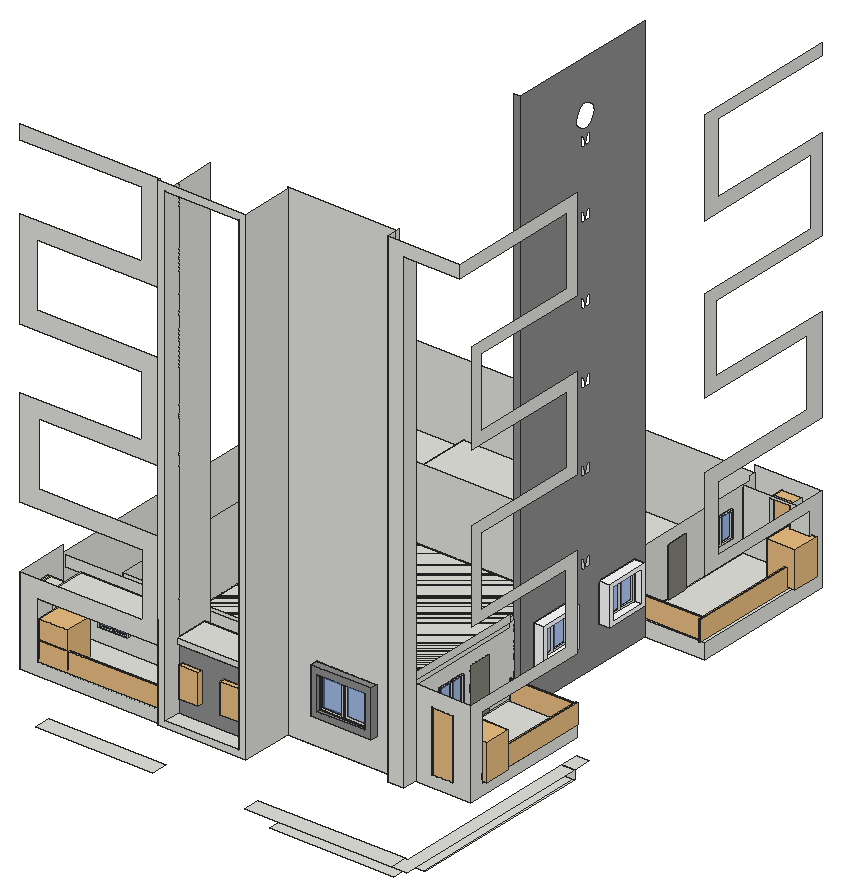
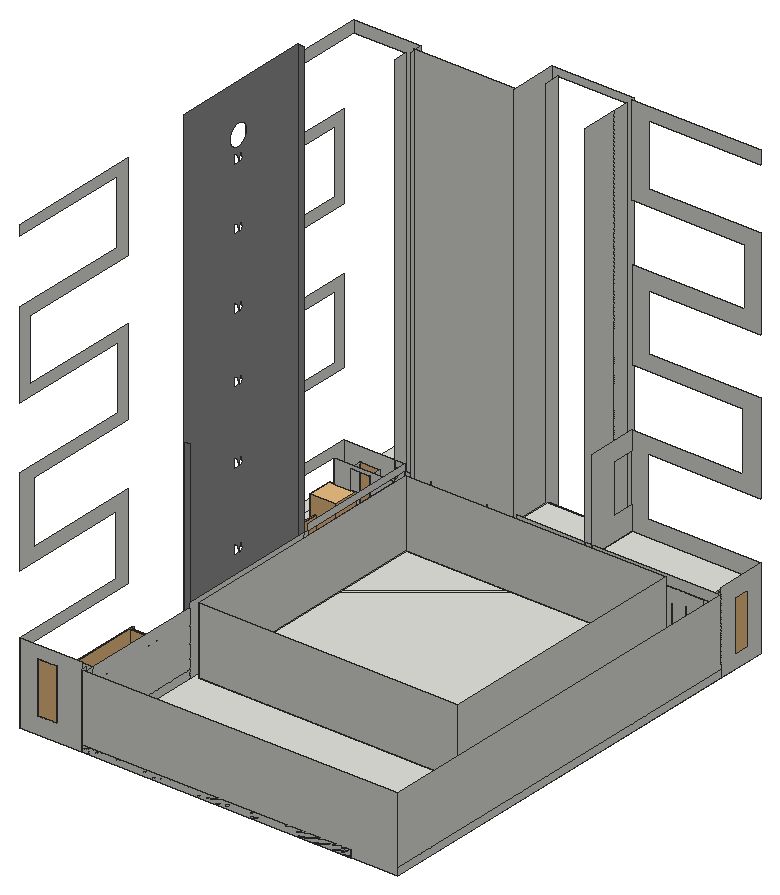
# SketchUp Ruby script. Lengths in inches.
U = 1.inch
M = Sketchup.active_model
def pt(a) = Geom::Point3d.new(a.map { |v| v * U })
def face(e, loops, mat)
  f = e.add_face(loops[0].map { |a| pt(a) })
  loops[1..].each { |l| e.add_face(l.map { |a| pt(a) }).erase! }
  f.material = f.back_material = mat if mat
  f
end
# faces: each face lists its corners as indices into pts; further lists are holes
def faces(e, pts, list, mat = nil) = list.each { |f| face(e, (f[0].is_a?(Array) ? f : [f]).map { |l| l.map { |i| pts[i] } }, mat) }
# xy, xz, yz: faces in a plane at the given z, y or x. An outline is a flat list of corners, or four numbers for a rectangle; further outlines are holes
def ring(l) = l.size == 4 ? [[l[0], l[1]], [l[2], l[1]], [l[2], l[3]], [l[0], l[3]]] : l.each_slice(2).to_a
def flat(e, list, mat, &to3) = list.each { |f| face(e, (f[0].is_a?(Array) ? f : [f]).map { |l| ring(l).map { |u, v| to3.(u, v) } }, mat) }
def xy(e, z, list, mat = nil) = flat(e, list, mat) { |x, y| [x, y, z] }
def xz(e, y, list, mat = nil) = flat(e, list, mat) { |x, z| [x, y, z] }
def yz(e, x, list, mat = nil) = flat(e, list, mat) { |y, z| [x, y, z] }
def lines(e, pts, list) = list.each { |a, b| e.add_line(pt(pts[a]), pt(pts[b])) }
# prism: a flat outline (further loops are holes) pulled along v
def prism(e, loops, v, mat = nil)
  f = face(e, loops, mat); d = Geom::Vector3d.new(v.map { |x| x * U })
  f.pushpull(f.normal.samedirection?(d) ? d.length : -d.length)
end
def box(e, o, s, mat = nil) = prism(e, [[o, [o[0] + s[0], o[1], o[2]], [o[0] + s[0], o[1] + s[1], o[2]], [o[0], o[1] + s[1], o[2]]]], [0, 0, s[2]], mat)
def at(x, y, z, deg = 0) = Geom::Transformation.translation(pt([x, y, z])) * Geom::Transformation.rotation(ORIGIN, Z_AXIS, deg.degrees)
def axes(o, x, y, z) = Geom::Transformation.new([*x, 0, *y, 0, *z, 0, *pt(o).to_a, 1])
def part(name) = M.definitions.add(name)
# library, detail: a bought-in or finely detailed component or shape, given as its bounding box
def library(name, o, s) = part(name).tap { |d| box(d.entities, o, s) }
def detail(e, o, s) = box(e.add_group.entities, o, s)
def put(e, d, t, mat = nil) = e.add_instance(d, t).tap { |i| i.material = mat if mat }
def group(e, t, mat = nil) = e.add_group.tap { |g| g.transformation = t; g.material = mat if mat }.entities
root = M.entities
M.materials.add("[Color M00]").color = [255, 255, 255]
M.materials.add("[Color M04]").color = [142, 142, 142]
M.materials.add("[Translucent Glass Blue]").color = [100, 149, 237]
M.materials["[Translucent Glass Blue]"].alpha = 0.5
M.materials.add("pic").color = [134, 132, 121]
c1 = library("grade+varanda",[25.2,-1.57,0],[92.91,3.14,40.94])
c2 = library("CNC CUTTING TEXTURE",[0,0,-0.79],[85.98,295.47,0.79])
c3 = part("Door leaf")
xy(c3.entities,0,[[0,0,28.74,2]],"pic")
xy(c3.entities,75.2,[[0,0,28.74,2]],"pic")
xz(c3.entities,0,[[0,0,28.74,75.2]],"pic")
xz(c3.entities,2,[[0,0,28.74,75.2]],"pic")
yz(c3.entities,0,[[0,0,2,75.2]])
yz(c3.entities,28.74,[[0,0,2,75.2]])
c4 = library("KentiaPalm",[-22.86,-14.31,0],[47.49,43.96,59.125])
c5 = library("Framed window",[0,0,0],[23.62,8.27,35.43])
c6 = part("Janela aluminio")
xy(c6.entities,0,[[0,0,47.24,1.57],[23.62,1.57,47.24,2.76],[0,2.76,25.98,3.9375],[0,3.9375,47.24,5.91]])
xy(c6.entities,43.31,[[0,0,47.24,1.57],[23.62,1.57,47.24,2.76],[0,2.76,0,5.91,47.24,5.91,47.24,3.9375,25.98,3.9375,25.98,2.76],[25.98,2.76,47.24,3.9375]])
xz(c6.entities,1.57,[[0,0,23.62,0,23.62,41.34,21.26,41.34,21.26,1.97,1.97,1.97,1.97,41.34,23.62,41.34,23.62,43.31,0,43.31],[[23.62,0,47.24,43.31],[25.7,1.97,45.28,41.34]]])
xz(c6.entities,2.76,[[[0,0,23.62,43.31],[2.36,2.36,21.26,40.94]],[23.62,0,25.98,43.31]])
xz(c6.entities,2.76,[[2.36,2.36,21.26,40.94]],"[Translucent Glass Blue]")
xz(c6.entities,3.9375,[[25.98,0,25.98,2.36,44.88,2.36,44.88,40.94,25.98,40.94,25.98,43.31,47.24,43.31,47.24,0]])
xz(c6.entities,3.9375,[[25.98,2.36,44.88,40.94]],"[Translucent Glass Blue]")
yz(c6.entities,0,[[0,0,1.57,43.31],[2.76,0,5.91,43.31]])
yz(c6.entities,23.62,[[1.57,0,2.76,43.31]])
yz(c6.entities,25.98,[[2.76,0,3.9375,43.31]])
yz(c6.entities,47.24,[[0,0,1.57,43.31],[1.57,0,2.76,43.31],[3.9375,0,5.91,43.31]])
c7 = part("Group\#81")
xy(c7.entities,0,[[[0,0,99.375,76.3125],[10.74,10.74,88.63,65.57]],[10.74,10.74,88.63,65.57]])
xy(c7.entities,11.8125,[[[0,0,99.375,76.3125],[10.74,10.74,88.63,65.57]]])
xz(c7.entities,0,[[0,0,99.375,11.8125]])
xz(c7.entities,10.74,[[10.74,0,88.63,11.8125]])
xz(c7.entities,65.57,[[10.74,0,88.63,11.8125]])
xz(c7.entities,76.3125,[[0,0,99.375,11.8125]])
yz(c7.entities,0,[[0,0,76.3125,11.8125]])
yz(c7.entities,10.74,[[10.74,0,65.57,11.8125]])
yz(c7.entities,88.63,[[10.74,0,65.57,11.8125]])
yz(c7.entities,99.375,[[0,0,76.3125,11.8125]])
c8 = part("Group\#73")
xy(c8.entities,0,[[6.22,6.22,66.16,57.66]],"[Color M00]")
xy(c8.entities,0,[[[0,0,72.375,63.875],[6.22,6.22,66.16,57.66]]],"[Color M04]")
xy(c8.entities,16.6875,[[[0,0,72.375,63.875],[6.22,6.22,66.16,57.66]]],"[Color M00]")
xz(c8.entities,0,[[0,0,72.375,16.6875]],"[Color M00]")
xz(c8.entities,6.22,[[6.22,0,66.16,16.6875]],"[Color M00]")
xz(c8.entities,57.66,[[6.22,0,66.16,16.6875]],"[Color M04]")
xz(c8.entities,63.875,[[0,0,72.375,16.6875]],"[Color M00]")
yz(c8.entities,0,[[0,0,63.875,16.6875]],"[Color M00]")
yz(c8.entities,6.22,[[6.22,0,57.66,16.6875]],"[Color M00]")
yz(c8.entities,66.16,[[6.22,0,57.66,16.6875]],"[Color M00]")
yz(c8.entities,72.375,[[0,0,63.875,16.6875]],"[Color M00]")
xy(root,159.08,[[[571.01,129.69,571.01,222.13,436.38,222.13,436.38,133.63,206.95,133.63,206.95,942.88,769.63,942.88,769.63,222.13,759.63,222.13,759.63,214.57,582.45,214.57,582.45,129.69],[298.63,231.13,760.63,693.13]],[436.38,129.69,571.01,222.13],[759.63,198.76,759.63,222.13,769.63,222.13,769.63,221.79,787.51,221.79,787.51,198.76],[769.63,221.79,787.51,222.13],[787.51,221.79,787.51,222.13,769.63,222.13,769.63,439.19,879.32,439.19,879.32,221.79],
  [769.63,447.18,780.63,702.13],[769.63,702.13,879.32,942.88]])
xy(root,163.67,[[929.91,38.75,947.1,345.07],[947.1,38.75,950.48,345.07]])
xy(root,166.08,[[725.85,0,929.91,27.4375]])
xy(root,169.09,[[448.85,129.69,571.01,157.26]])
xy(root,171.08,[[298.63,231.13,760.63,693.13]])
xy(root,178.14,[[769.63,244.2,879.32,439.19]])
xy(root,178.33,[[815.15,221.79,849.53,244.2]])
xy(root,179.08,[[340.16,0,532.72,27.4375],[683.66,0,925.48,27.4375],[925.48,0,950.48,0,950.48,345.07,929.91,345.07,929.91,27.4375,925.48,27.4375],[929.91,345.07,950.48,374.76]])
xy(root,180.77,[[236.76,133.63,436.38,222.13]])
xy(root,182.11,[[206.95,161.73,236.76,191.1]])
xy(root,183.96,[[769.63,702.13,879.32,917.62]])
xy(root,190.29,[[813.66,917.62,847.23,942.88]])
xy(root,272.74,[[206.95,161.73,236.76,191.1]])
xy(root,273.03,[[448.85,157.26,571.01,210.63]],"[Color M04]")
xy(root,273.46,[[236.76,133.63,436.38,222.13]])
xz(root,129.69,[[[436.38,159.08,582.45,963.08],[448.85,169.09,571.01,951.08]]])
xz(root,133.63,[[206.95,159.08,436.38,159.08,436.38,180.77,236.76,180.77,236.76,273.46,436.38,273.46,436.38,435.08,237.95,435.08,237.95,538.83,435.45,538.83,435.45,699.08,234.54,699.08,234.54,802.33,436.38,802.33,436.38,963.08,206.95,963.08,206.95,939.77,406.75,939.77,406.75,831.08,206.95,831.08,206.95,667.96,406.86,667.96,406.86,567.08,206.95,567.08,206.95,406.33,408.57,406.33,408.57,303.08,206.95,303.08]])
xz(root,157.26,[[448.85,169.09,571.01,273.03]],"[Color M04]")
xz(root,161.73,[[206.95,182.11,236.76,272.74]])
xz(root,191.1,[[206.95,182.11,236.76,272.74]])
xz(root,198.76,[[759.63,159.08,787.51,159.08,787.51,942.33,879.32,942.33,879.32,963.08,759.63,963.08]])
xz(root,214.57,[[582.45,159.08,759.63,966.02]])
xz(root,221.79,[[[769.63,159.08,879.32,303.08],[815.15,178.33,849.53,277.65]]])
xz(root,222.13,[[436.38,159.08,571.01,159.08,571.01,169.09,448.85,169.09,448.85,291.08,436.38,291.08],[759.63,159.08,769.63,291.08],[769.63,159.08,787.51,171.08],[448.85,169.09,571.01,291.08],[769.63,171.08,787.51,291.08],
  [236.76,180.77,436.38,273.46],[211.74,273.46,436.38,291.08]])
xz(root,231.13,[[298.63,159.08,760.63,171.08],[298.63,171.08,760.63,291.08]])
xz(root,244.2,[[[769.63,178.14,879.32,284.02],[815.15,178.33,849.53,277.65]]])
xz(root,345.07,[[929.91,163.67,950.48,179.08]])
xz(root,439.19,[[769.63,159.08,879.32,178.14]])
xz(root,447.18,[[769.63,159.08,780.63,1067.71]],"[Color M04]")
xz(root,693.13,[[298.63,159.08,760.63,171.08],[298.63,171.08,760.63,291.08]])
xz(root,702.13,[[780.63,159.08,879.32,183.96]])
xz(root,702.13,[[769.63,183.96,780.63,545.21]],"[Color M04]")
xz(root,917.62,[[[769.63,183.96,879.32,283.71],[813.66,190.29,847.23,281.29]]])
xz(root,942.88,[[206.95,159.08,769.63,291.08],[[769.63,159.08,879.32,303.08],[813.66,190.29,847.23,281.29]]])
yz(root,206.95,[[[133.63,159.08,222.13,303.08],[161.73,182.11,191.1,272.74]],[222.13,159.08,942.88,171.08],[222.13,171.08,942.88,291.08]])
yz(root,236.76,[[[133.63,180.77,222.13,273.46],[161.73,182.11,191.1,272.74]]])
yz(root,298.63,[[231.13,159.08,693.13,171.08],[231.13,171.08,693.13,291.08]])
yz(root,436.38,[[129.69,159.08,133.63,180.77],[133.63,159.08,222.13,180.77],[129.69,180.77,222.13,273.46],[129.69,273.46,133.63,315.48],[133.63,273.46,222.13,273.46,222.13,435.08,133.63,435.08,133.63,402.1,173.48,402.1,173.48,315.48,133.63,315.48]])
yz(root,448.85,[[129.69,169.09,157.26,169.09,157.26,273.03,210.63,273.03,210.63,281.18,157.26,281.18,157.26,951.08,129.69,951.08],[157.26,169.09,222.13,169.09,222.13,951.08,157.26,951.08,157.26,281.18,210.63,281.18,210.63,273.03,157.26,273.03]])
yz(root,571.01,[[129.69,169.09,129.69,951.08,157.26,951.08,157.26,281.18,210.63,281.18,210.63,273.03,157.26,273.03,157.26,169.09]])
yz(root,582.45,[[129.69,159.08,214.57,963.08]])
yz(root,759.63,[[198.76,159.08,214.57,963.08],[214.57,159.08,222.13,963.08]])
yz(root,760.63,[[231.13,159.08,693.13,171.08],[231.13,171.08,693.13,291.08]])
yz(root,769.63,[[221.79,159.08,221.79,303.08,439.19,303.08,439.19,291.08,222.13,291.08,222.13,159.08],[222.13,159.08,238.89,159.08,238.89,178.14,244.2,178.14,244.2,287.21,238.89,287.21,238.89,291.08,222.13,291.08],[238.89,159.08,439.19,178.14],[439.19,159.08,447.18,159.08,447.18,291.08,439.19,291.08,439.19,284.02,244.2,284.02,244.2,178.14,439.19,178.14],[447.18,159.08,702.13,159.08,702.13,283.71,702.05,283.71,702.05,291.08,447.18,291.08],
  [702.13,159.08,917.62,183.96],[917.62,159.08,942.88,159.08,942.88,291.08,933.12,291.08,933.12,283.71,917.62,283.71],[702.13,183.96,917.62,283.71]])
yz(root,780.63,[[[447.18,159.08,702.13,159.08,702.13,283.71,702.05,283.71,702.05,435.08,702.13,435.08,702.13,1067.71,447.18,1067.71],[579.22,962.375,574.32,963.14,569.78,965.15,565.92,968.27,563,972.27,561.22,976.9,560.6875,981.83,561.46,986.73,563.47,991.27,566.58,995.13,570.59,998.05,575.22,999.84,580.15,1000.36,585.05,999.6,589.58,997.59,593.44,994.47,596.36,990.46,598.15,985.84,598.68,980.9,597.91,976,595.9,971.47,592.79,967.61,588.78,964.6875,584.15,962.9],[587.71,936.74,586.81,936.76,585.85,936.8,584.98,936.91,584.45,936.78,582.77,937.01,581.3,938,579.62,939.54,579.78,942.57,579.83,943.35,579.89,944.06,579.97,944.99,580.16,945.91,580.27,946.81,580.42,947.6875,580.71,948.53,581.12,949.24,581.45,949.95,581.94,950.63,582.55,951.1,583.01,951.79,583.98,952.52,584.71,952.93,585.43,953.4375,586.15,953.85,586.76,954.35,587.47,954.72,588.13,955.25,588.79,955.63,589.35,955.7,589.65,955.95,589.56,955.375,589.55,954.46,589.56,953.53,589.59,952.61,589.63,951.8,589.7,950.88,590.03,949.89,590.03,949.13,590.13,948.35,590.11,947.57,590.09,946.86,590.07,945.91,590.04,944.97,590.01,944.13,589.97,943.07,589.91,942.15,589.84,941.32,589.71,940.31,589.55,939.4375,589.32,938.61,588.74,937.97,588.31,937.29],[587.71,825.49,586.81,825.51,585.85,825.55,584.98,825.66,584.45,825.53,582.77,825.76,581.3,826.75,579.62,828.29,579.78,831.32,579.83,832.1,579.89,832.81,579.97,833.74,580.16,834.66,580.27,835.56,580.42,836.4375,580.71,837.28,581.12,837.99,581.45,838.7,581.94,839.38,582.55,839.85,583.01,840.54,583.98,841.27,584.71,841.68,585.43,842.1875,586.15,842.6,586.76,843.1,587.47,843.47,588.13,844,588.79,844.38,589.35,844.45,589.65,844.7,589.56,844.125,589.55,843.21,589.56,842.28,589.59,841.36,589.63,840.55,589.7,839.63,590.03,838.64,590.03,837.88,590.13,837.1,590.11,836.32,590.09,835.61,590.07,834.66,590.04,833.72,590.01,832.88,589.97,831.82,589.91,830.9,589.84,830.07,589.71,829.06,589.55,828.1875,589.32,827.36,588.74,826.72,588.31,826.04],[587.71,698.18,586.81,698.19,585.85,698.24,584.98,698.34,584.45,698.22,582.77,698.45,581.3,699.43,579.62,700.97,579.78,704,579.83,704.79,579.89,705.5,579.97,706.43,580.16,707.35,580.27,708.25,580.42,709.125,580.71,709.97,581.12,710.68,581.45,711.38,581.94,712.07,582.55,712.54,583.01,713.23,583.98,713.96,584.71,714.37,585.43,714.875,586.15,715.28,586.76,715.79,587.47,716.16,588.13,716.6875,588.79,717.07,589.35,717.14,589.65,717.39,589.56,716.8125,589.55,715.89,589.56,714.97,589.59,714.05,589.63,713.24,589.7,712.32,590.03,711.33,590.03,710.57,590.13,709.79,590.11,709,590.09,708.3,590.07,707.35,590.04,706.41,590.01,705.57,589.97,704.51,589.91,703.59,589.84,702.76,589.71,701.75,589.55,700.875,589.32,700.05,588.74,699.41,588.31,698.73],[587.71,581.05,586.81,581.07,585.85,581.11,584.98,581.22,584.45,581.1,582.77,581.32,581.3,582.31,579.62,583.85,579.78,586.88,579.83,587.66,579.89,588.37,579.97,589.3,580.16,590.22,580.27,591.12,580.42,592,580.71,592.85,581.12,593.55,581.45,594.26,581.94,594.94,582.55,595.42,583.01,596.11,583.98,596.84,584.71,597.25,585.43,597.75,586.15,598.16,586.76,598.66,587.47,599.03,588.13,599.5625,588.79,599.95,589.35,600.01,589.65,600.27,589.56,599.6875,589.55,598.77,589.56,597.85,589.59,596.93,589.63,596.12,589.7,595.2,590.03,594.2,590.03,593.44,590.13,592.66,590.11,591.88,590.09,591.17,590.07,590.22,590.04,589.29,590.01,588.44,589.97,587.39,589.91,586.46,589.84,585.63,589.71,584.62,589.55,583.75,589.32,582.92,588.74,582.28,588.31,581.6],[587.71,450.99,586.81,451.01,585.85,451.05,584.98,451.16,584.45,451.03,582.77,451.26,581.3,452.25,579.62,453.79,579.78,456.82,579.83,457.6,579.89,458.31,579.97,459.24,580.16,460.16,580.27,461.06,580.42,461.9375,580.71,462.78,581.12,463.49,581.45,464.2,581.94,464.88,582.55,465.35,583.01,466.04,583.98,466.77,584.71,467.18,585.43,467.6875,586.15,468.1,586.76,468.6,587.47,468.97,588.13,469.5,588.79,469.88,589.35,469.95,589.65,470.2,589.56,469.625,589.55,468.71,589.56,467.78,589.59,466.86,589.63,466.05,589.7,465.13,590.03,464.14,590.03,463.38,590.13,462.6,590.11,461.82,590.09,461.11,590.07,460.16,590.04,459.22,590.01,458.38,589.97,457.32,589.91,456.4,589.84,455.57,589.71,454.56,589.55,453.6875,589.32,452.86,588.74,452.22,588.31,451.54],[587.71,313.43,586.81,313.44,585.85,313.49,584.98,313.59,584.45,313.47,582.77,313.7,581.3,314.68,579.62,316.22,579.78,319.25,579.83,320.04,579.89,320.75,579.97,321.68,580.16,322.6,580.27,323.5,580.42,324.375,580.71,325.22,581.12,325.93,581.45,326.63,581.94,327.32,582.55,327.79,583.01,328.48,583.98,329.21,584.71,329.62,585.43,330.125,586.15,330.53,586.76,331.04,587.47,331.41,588.13,331.9375,588.79,332.32,589.35,332.39,589.65,332.64,589.56,332.0625,589.55,331.14,589.56,330.22,589.59,329.3,589.63,328.49,589.7,327.57,590.03,326.58,590.03,325.82,590.13,325.04,590.11,324.25,590.09,323.55,590.07,322.6,590.04,321.66,590.01,320.82,589.97,319.76,589.91,318.84,589.84,318.01,589.71,317,589.55,316.125,589.32,315.3,588.74,314.66,588.31,313.98],[577.58,824.8125,576.67,824.89,575.7,825.01,574.95,825.17,574.125,825.39,573.44,825.88,572.79,826.49,572.09,826.95,571.66,827.83,571.28,828.61,571.05,829.39,570.87,830.1,570.9375,831.01,571.01,831.85,571.1,832.86,571.36,833.57,571.5,834.68,571.52,835.45,571.54,836.21,571.55,837.05,571.52,837.85,571.63,838.48,571.5,840.17,571,841.86,571.06,843.72,572.6875,843.14,572.95,842.58,573.76,842.29,574.43,841.66,575.21,840.99,575.73,840.54,576.3,839.86,576.64,839.16,576.92,838.34,577.16,837.48,577.48,836.81,577.81,836.05,577.92,835.29,577.98,834.3125,578.03,833.51,578.04,832.61,578.04,831.79,578.48,831.11,578.67,830.34,579.62,828.29,579.45,827.42,579.23,826.6,578.83,825.88,578.17,825.34],[577.58,697.5,576.67,697.57,575.7,697.69,574.95,697.86,574.125,698.07,573.44,698.57,572.79,699.18,572.09,699.64,571.66,700.52,571.28,701.3,571.05,702.08,570.87,702.79,570.9375,703.7,571.01,704.54,571.1,705.55,571.36,706.26,571.5,707.37,571.52,708.14,571.54,708.9,571.55,709.74,571.52,710.54,571.63,711.16,571.5,712.85,571,714.54,571.06,716.41,572.6875,715.83,572.95,715.27,573.76,714.98,574.43,714.35,575.21,713.68,575.73,713.23,576.3,712.55,576.64,711.85,576.92,711.03,577.16,710.16,577.48,709.49,577.81,708.73,577.92,707.97,577.98,707,578.03,706.2,578.04,705.29,578.04,704.48,578.48,703.8,578.67,703.03,579.62,700.97,579.45,700.11,579.23,699.29,578.83,698.56,578.17,698.03],[577.58,580.375,576.67,580.45,575.7,580.57,574.95,580.73,574.125,580.95,573.44,581.44,572.79,582.05,572.09,582.51,571.66,583.4,571.28,584.18,571.05,584.95,570.87,585.67,570.9375,586.58,571.01,587.41,571.1,588.42,571.36,589.13,571.5,590.24,571.52,591.01,571.54,591.77,571.55,592.62,571.52,593.42,571.63,594.04,571.5,595.73,571,597.42,571.06,599.29,572.6875,598.71,572.95,598.14,573.76,597.85,574.43,597.22,575.21,596.56,575.73,596.1,576.3,595.43,576.64,594.73,576.92,593.91,577.16,593.04,577.48,592.37,577.81,591.61,577.92,590.85,577.98,589.875,578.03,589.07,578.04,588.17,578.04,587.35,578.48,586.67,578.67,585.9,579.62,583.85,579.45,582.99,579.23,582.16,578.83,581.44,578.17,580.9],[577.58,450.3125,576.67,450.39,575.7,450.51,574.95,450.67,574.125,450.89,573.44,451.38,572.79,451.99,572.09,452.45,571.66,453.33,571.28,454.11,571.05,454.89,570.87,455.6,570.9375,456.51,571.01,457.35,571.1,458.36,571.36,459.07,571.5,460.18,571.52,460.95,571.54,461.71,571.55,462.55,571.52,463.35,571.63,463.98,571.5,465.67,571,467.36,571.06,469.22,572.6875,468.64,572.95,468.08,573.76,467.79,574.43,467.16,575.21,466.49,575.73,466.04,576.3,465.36,576.64,464.66,576.92,463.84,577.16,462.98,577.48,462.31,577.81,461.55,577.92,460.79,577.98,459.8125,578.03,459.01,578.04,458.11,578.04,457.29,578.48,456.61,578.67,455.84,579.62,453.79,579.45,452.92,579.23,452.1,578.83,451.38,578.17,450.84],[577.58,312.75,576.67,312.82,575.7,312.94,574.95,313.11,574.125,313.32,573.44,313.82,572.79,314.43,572.09,314.89,571.66,315.77,571.28,316.55,571.05,317.33,570.87,318.04,570.9375,318.95,571.01,319.79,571.1,320.8,571.36,321.51,571.5,322.62,571.52,323.39,571.54,324.15,571.55,324.99,571.52,325.79,571.63,326.41,571.5,328.1,571,329.79,571.06,331.66,572.6875,331.08,572.95,330.52,573.76,330.23,574.43,329.6,575.21,328.93,575.73,328.48,576.3,327.8,576.64,327.1,576.92,326.28,577.16,325.41,577.48,324.74,577.81,323.98,577.92,323.22,577.98,322.25,578.03,321.45,578.04,320.54,578.04,319.73,578.48,319.05,578.67,318.28,579.62,316.22,579.45,315.36,579.23,314.54,578.83,313.81,578.17,313.28],[577.58,936.0625,576.67,936.14,575.7,936.26,574.95,936.42,574.125,936.64,573.44,937.13,572.79,937.74,572.09,938.2,571.66,939.08,571.28,939.86,571.05,940.64,570.87,941.35,570.9375,942.26,571.01,943.1,571.1,944.11,571.36,944.82,571.5,945.93,571.52,946.7,571.54,947.46,571.55,948.3,571.52,949.1,571.63,949.73,571.5,951.42,571,953.11,571.06,954.97,572.6875,954.39,572.95,953.83,573.76,953.54,574.43,952.91,575.21,952.24,575.73,951.79,576.3,951.11,576.64,950.41,576.92,949.59,577.16,948.73,577.48,948.06,577.81,947.3,577.92,946.54,577.98,945.5625,578.03,944.76,578.04,943.86,578.04,943.04,578.48,942.36,578.67,941.59,579.62,939.54,579.45,938.67,579.23,937.85,578.83,937.13,578.17,936.59],[589.65,955.95,589.67,956.08,591.45,958.31,590.67,956.82],[589.65,844.7,589.67,844.83,591.45,847.06,590.67,845.57],[589.65,717.39,589.67,717.52,591.45,719.75,590.67,718.25],[589.65,600.27,589.67,600.39,591.45,602.62,590.67,601.13],[589.65,470.2,589.67,470.33,591.45,472.56,590.67,471.07],[589.65,332.64,589.67,332.77,591.45,335,590.67,333.5]]],"[Color M04]")
yz(root,787.51,[[198.76,159.08,222.13,942.33]])
yz(root,813.66,[[917.62,190.29,942.88,281.29]])
yz(root,815.15,[[221.79,178.33,244.2,277.65]])
yz(root,847.23,[[917.62,190.29,942.88,281.29]])
yz(root,849.53,[[221.79,178.33,244.2,277.65]])
yz(root,879.32,[[221.79,159.08,439.19,159.08,439.19,178.14,244.2,178.14,244.2,284.02,439.19,284.02,439.19,435.08,242.1,435.08,242.1,548.14,439.19,548.14,439.19,699.08,242.375,699.08,242.375,812.14,439.19,812.14,439.19,963.08,198.76,963.08,198.76,942.33,419.01,942.33,419.01,831.08,222.13,831.08,222.13,679.46,418.66,679.46,418.66,567.08,222.13,567.08,222.13,418.39,415.6,418.39,415.6,303.08,221.79,303.08],[702.13,159.08,942.88,159.08,942.88,303.08,728.91,303.08,728.91,410.02,942.88,410.02,942.88,567.08,725.74,567.08,725.74,678.39,942.88,678.39,942.88,831.08,728.37,831.08,728.37,944.96,942.88,944.96,942.88,963.08,702.13,963.08,702.13,807.39,921.54,807.39,921.54,699.08,702.13,699.08,702.13,545.21,913.11,545.21,913.11,435.08,702.13,435.08,702.13,283.71,917.62,283.71,917.62,183.96,702.13,183.96]])
g1 = group(root,at(289.63,702.13,159.08))
box(g1,[0,-480,0],[480,720.75,12])
put(root,c1,axes([744,436.22,178.12],[1.0998,0,0],[0,1,0],[0,0,0.8]))
put(root,c1,axes([877.75,190.78,178.3125],[0,2.12,0],[-1,0,0],[0,0,0.8]))
put(root,c2,axes([816.04,221.79,178.33],[0.3894,0,0],[0,0,0.33611],[0,-1.1913,0]))
put(root,c1,axes([183.35,135.21,180.7],[2.12,0,0],[0,1,0],[0,0,0.8]))
put(root,c1,axes([431.96,244.65,180.77],[0.02789,-0.93959,0],[0.99956,0.02967,0],[0,0,0.8]))
put(root,c3,axes([367.18,217.42,180.77],[1.26,0,0],[0,1,0],[0,0,1.1]))
put(root,c3,axes([771.63,355.51,181.79],[0,1.26,0],[-1,0,0],[0,0,1.1]))
put(root,c3,axes([771.63,762.45,181.79],[0,1.26,0],[-1,0,0],[0,0,1.1]))
put(root,c2,axes([206.95,161.52,182.11],[0,0.34407,0],[0,0,0.30671],[-6.34963,0,0]))
put(root,c4,at(863.43,257.21,182.83))
put(root,c1,axes([742.6,707.43,183.96],[1.0998,0,0],[0,1,0],[0,0,0.8]))
put(root,c1,axes([872.12,642.18,183.96],[0,2.332,0],[-1,0,0],[0,0,0.8]))
put(root,c4,at(260.75,149,185.11))
put(root,c4,at(863.43,891.72,188.19))
put(root,c2,axes([813.74,942.88,190.29],[0.3894,0,0],[0,0,0.30798],[0,19.75175,0]))
put(root,c5,axes([529.875,141.71,201.71],[1.35,0,0],[0,1,0],[0,0,1.38]))
put(root,c5,axes([461.6875,141.71,201.71],[1.35,0,0],[0,1,0],[0,0,1.38]))
put(root,c6,at(269.17,216.22,206.77))
put(root,c7,axes([630.14,214.57,207.85],[1,0,0],[0,0,1],[0,-1,0]),"[Color M04]")
put(root,c8,axes([780.82,472.87,216.18],[0,1,0],[0,0,1],[1,0,0]),"[Color M00]")
put(root,c6,at(774.2,290.89,217.36,90))
put(root,c6,at(774.2,845.05,217.36,90))
put(root,c8,axes([780.63,608.66,218.72],[0,1,0],[0,0,1],[1,0,0]),"[Color M00]")
put(root,c6,axes([720.02,213.44,219.25],[-1.675,0,0],[0,-1,0],[0,0,1.25072]))
put(root,c6,axes([785.51,479.08,222.39],[0,1.25,0],[-1,0,0],[0,0,1.1998]))
put(root,c6,axes([786.92,614.88,224.9375],[0,1.25,0],[-1,0,0],[0,0,1.1998]))
g2 = group(root,at(448.85,210.63,273.03))
box(g2,[0,-57.1875,0],[122.16,57.1875,8.15])
